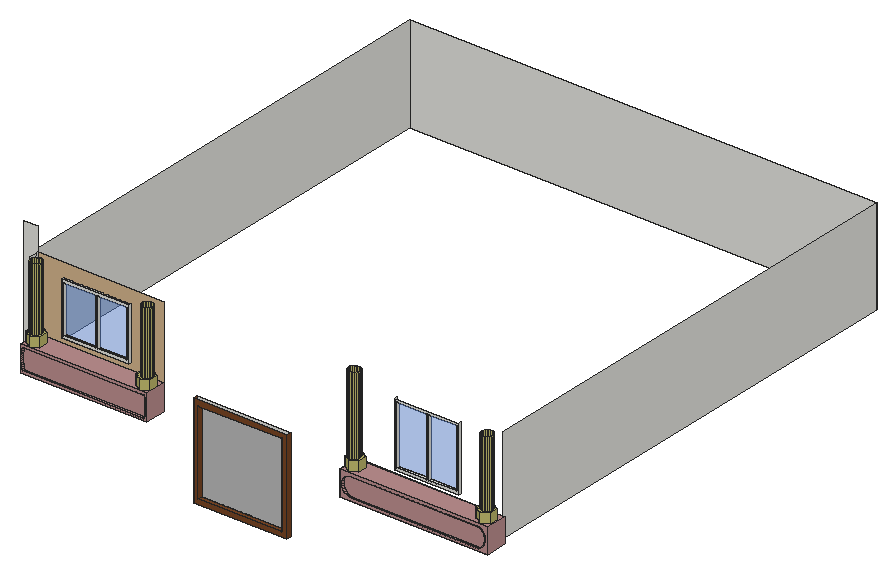
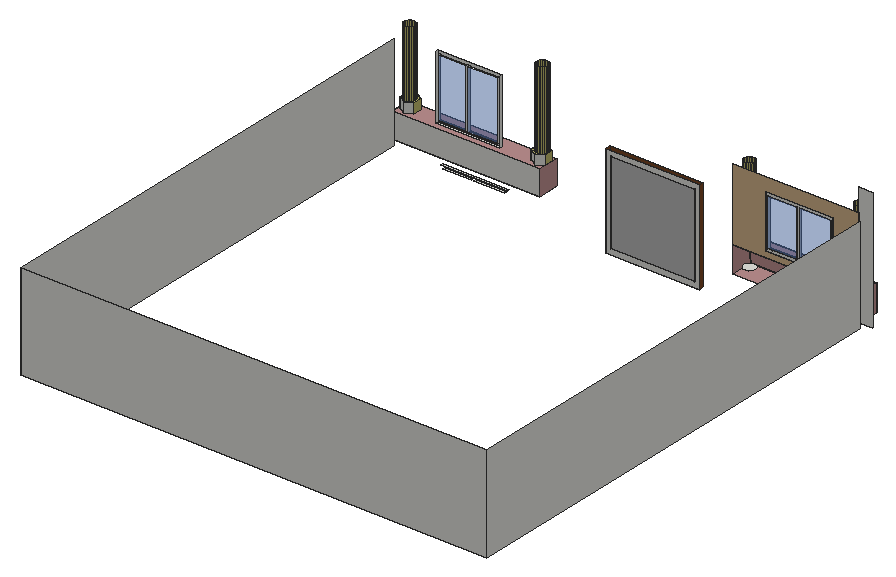
# SketchUp Ruby script. Lengths in inches.
U = 1.inch
M = Sketchup.active_model
def pt(a) = Geom::Point3d.new(a.map { |v| v * U })
def face(e, loops, mat)
  f = e.add_face(loops[0].map { |a| pt(a) })
  loops[1..].each { |l| e.add_face(l.map { |a| pt(a) }).erase! }
  f.material = f.back_material = mat if mat
  f
end
# faces: each face lists its corners as indices into pts; further lists are holes
def faces(e, pts, list, mat = nil) = list.each { |f| face(e, (f[0].is_a?(Array) ? f : [f]).map { |l| l.map { |i| pts[i] } }, mat) }
# xy, xz, yz: faces in a plane at the given z, y or x. An outline is a flat list of corners, or four numbers for a rectangle; further outlines are holes
def ring(l) = l.size == 4 ? [[l[0], l[1]], [l[2], l[1]], [l[2], l[3]], [l[0], l[3]]] : l.each_slice(2).to_a
def flat(e, list, mat, &to3) = list.each { |f| face(e, (f[0].is_a?(Array) ? f : [f]).map { |l| ring(l).map { |u, v| to3.(u, v) } }, mat) }
def xy(e, z, list, mat = nil) = flat(e, list, mat) { |x, y| [x, y, z] }
def xz(e, y, list, mat = nil) = flat(e, list, mat) { |x, z| [x, y, z] }
def yz(e, x, list, mat = nil) = flat(e, list, mat) { |y, z| [x, y, z] }
def lines(e, pts, list) = list.each { |a, b| e.add_line(pt(pts[a]), pt(pts[b])) }
# prism: a flat outline (further loops are holes) pulled along v
def prism(e, loops, v, mat = nil)
  f = face(e, loops, mat); d = Geom::Vector3d.new(v.map { |x| x * U })
  f.pushpull(f.normal.samedirection?(d) ? d.length : -d.length)
end
def box(e, o, s, mat = nil) = prism(e, [[o, [o[0] + s[0], o[1], o[2]], [o[0] + s[0], o[1] + s[1], o[2]], [o[0], o[1] + s[1], o[2]]]], [0, 0, s[2]], mat)
def at(x, y, z, deg = 0) = Geom::Transformation.translation(pt([x, y, z])) * Geom::Transformation.rotation(ORIGIN, Z_AXIS, deg.degrees)
def axes(o, x, y, z) = Geom::Transformation.new([*x, 0, *y, 0, *z, 0, *pt(o).to_a, 1])
def part(name) = M.definitions.add(name)
# library, detail: a bought-in or finely detailed component or shape, given as its bounding box
def library(name, o, s) = part(name).tap { |d| box(d.entities, o, s) }
def detail(e, o, s) = box(e.add_group.entities, o, s)
def put(e, d, t, mat = nil) = e.add_instance(d, t).tap { |i| i.material = mat if mat }
def group(e, t, mat = nil) = e.add_group.tap { |g| g.transformation = t; g.material = mat if mat }.entities
root = M.entities
M.materials.add("[0035_Tan]").color = [210, 180, 140]
M.materials.add("[0057_DarkKhaki]").color = [189, 183, 107]
M.materials.add("[0119_RosyBrown]").color = [188, 143, 143]
M.materials.add("[Mirror 01]").color = [185, 185, 185]
M.materials.add("[Translucent Glass Blue]").color = [100, 149, 237]
M.materials["[Translucent Glass Blue]"].alpha = 0.5
M.materials.add("[Wood Veneer 01]").color = [120, 70, 37]
xy(root,421.56,[[370.4,74.37,487.09,80.37]],"[Wood Veneer 01]")
xy(root,427.56,[[376.4,74.37,481.09,80.37]],"[Wood Veneer 01]")
xy(root,470.26,[[584.28,113.37,622.84,116.37],[626.17,113.37,661.4,116.37]])
xy(root,472.13,[[173.78,113.37,215.4,116.37],[217.84,113.37,257.03,116.37]])
xy(root,473.26,[[581.28,113.37,664.4,116.37]])
xy(root,475.13,[[170.78,113.37,260.03,116.37]])
xy(root,480,[[142.36,89.37,299.74,116.37]],"[0119_RosyBrown]")
xy(root,481.5,[[540.59,89.37,725.37,92.37],[540.59,92.37,725.37,116.37]],"[0119_RosyBrown]")
xy(root,483,[[145.36,89.37,296.74,92.37]],"[0119_RosyBrown]")
xy(root,484.5,[[711.84,99.06,713.26,99.24,714.59,99.79,715.73,100.67,716.6,101.81,717.15,103.13,717.34,104.56,717.15,105.98,716.6,107.31,715.73,108.44,714.59,109.32,713.26,109.87,711.84,110.06,710.41,109.87,709.09,109.32,707.95,108.44,707.07,107.31,706.53,105.98,706.34,104.56,706.53,103.13,707.07,101.81,707.95,100.67,709.09,99.79,710.41,99.24],[549.01,99.72,550.28,99.72,551.51,100.05,552.61,100.69,553.51,101.59,554.14,102.7,554.47,103.93,554.47,105.2,554.14,106.43,553.5,107.53,552.6,108.43,551.49,109.0625,550.26,109.39,548.99,109.39,547.76,109.06,546.66,108.42,545.76,107.52,545.13,106.41,544.8,105.19,544.8,103.91,545.13,102.68,545.77,101.58,546.67,100.68,547.78,100.05]])
xy(root,484.5,[[553.67,89.37,715.1,92.37]],"[0119_RosyBrown]")
xy(root,485.25,[[153.73,94.92,155.52,95.29,157.15,96.12,158.52,97.33,159.52,98.86,160.09,100.6,160.19,102.42,159.82,104.21,159,105.84,157.78,107.2,156.25,108.21,154.52,108.78,152.69,108.88,150.9,108.51,149.27,107.69,147.91,106.47,146.91,104.94,146.33,103.2,146.23,101.38,146.6,99.59,147.43,97.96,148.64,96.6,150.17,95.59,151.91,95.02],[289.98,96.17,291.77,96.54,293.4,97.37,294.77,98.58,295.77,100.11,296.34,101.85,296.44,103.67,296.07,105.46,295.25,107.09,294.03,108.45,292.5,109.46,290.77,110.03,288.94,110.13,287.15,109.76,285.52,108.94,284.16,107.72,283.16,106.19,282.58,104.45,282.48,102.63,282.85,100.84,283.68,99.21,284.89,97.85,286.42,96.84,288.16,96.27]])
xy(root,509.25,[[553.67,89.37,715.1,92.37]],"[0119_RosyBrown]")
xy(root,509.5625,[[145.36,89.37,296.74,92.37]],"[0119_RosyBrown]")
xy(root,512.25,[[[540.59,89.37,725.37,116.37],[550.07,91.65,541.14,96.81,541.14,107.12,550.07,112.27,559,107.12,559,96.81],[714.38,91.65,705.45,96.81,705.45,107.12,714.38,112.27,723.3125,107.12,723.3125,96.81]]],"[0119_RosyBrown]")
xy(root,512.5625,[[153.05,90.14,144.01,95.36,144.01,105.8,153.05,111.02,162.09,105.8,162.09,95.36],[290.49,90.14,281.45,95.36,281.45,105.8,290.49,111.02,299.53,105.8,299.53,95.36]])
xy(root,512.5625,[[[142.36,89.37,299.74,116.37],[290.49,90.14,281.45,95.36,281.45,105.8,290.49,111.02,299.53,105.8,299.53,95.36],[153.05,90.14,144.01,95.36,144.01,105.8,153.05,111.02,162.09,105.8,162.09,95.36]]],"[0119_RosyBrown]")
xy(root,518.48,[[590.68,113.37,670.37,116.37]])
xy(root,520.23,[[174.8,113.37,258.8,116.37]])
xy(root,521.48,[[593.68,113.37,630.53,116.37],[633.47,113.37,667.37,116.37]])
xy(root,523.23,[[177.8,113.37,216.8,116.37],[219.92,113.37,255.8,116.37]])
xy(root,524.25,[[[550.07,91.65,559,96.81,559,107.12,550.07,112.27,541.14,107.12,541.14,96.81],[548.88,95.41,547.09,95.64,545.41,96.33,543.98,97.4375,542.875,98.875,542.18,100.55,541.95,102.34,542.18,104.14,542.875,105.8125,543.98,107.25,545.41,108.35,547.09,109.04,548.88,109.28,550.68,109.04,552.35,108.35,553.79,107.25,554.89,105.8125,555.58,104.14,555.82,102.34,555.58,100.55,554.89,98.875,553.79,97.4375,552.35,96.33,550.68,95.64]],[[714.38,91.65,723.3125,96.81,723.3125,107.12,714.38,112.27,705.45,107.12,705.45,96.81],[714.7,95.41,712.9,95.64,711.23,96.33,709.79,97.4375,708.6875,98.875,707.99,100.55,707.76,102.34,707.99,104.14,708.6875,105.8125,709.79,107.25,711.23,108.35,712.9,109.04,714.7,109.28,716.49,109.04,718.16,108.35,719.6,107.25,720.7,105.8125,721.4,104.14,721.63,102.34,721.4,100.55,720.7,98.875,719.6,97.4375,718.16,96.33,716.49,95.64]]],"[0057_DarkKhaki]")
xy(root,524.5625,[[[153.05,90.14,162.09,95.36,162.09,105.8,153.05,111.02,144.01,105.8,144.01,95.36],[152.5,94.42,150.78,94.71,149.19,95.4375,147.84,96.55,146.83,97.97,146.22,99.61,146.06,101.35,146.35,103.07,147.07,104.66,148.18,106,149.61,107.01,151.24,107.625,152.98,107.79,154.7,107.5,156.29,106.77,157.64,105.66,158.65,104.24,159.26,102.6,159.42,100.87,159.13,99.14,158.41,97.56,157.3,96.21,155.875,95.2,154.24,94.59]],[[290.49,90.14,299.53,95.36,299.53,105.8,290.49,111.02,281.45,105.8,281.45,95.36],[291.4,94.48,289.68,94.66,288.07,95.28,286.67,96.3,285.58,97.65,284.88,99.23,284.61,100.93,284.79,102.65,285.41,104.27,286.42,105.67,287.77,106.76,289.35,107.46,291.06,107.73,292.78,107.55,294.39,106.93,295.79,105.91,296.88,104.57,297.58,102.99,297.85,101.28,297.67,99.56,297.05,97.95,296.04,96.55,294.69,95.46,293.11,94.75]]],"[0057_DarkKhaki]")
xz(root,74.37,[[[370.4,421.56,487.09,538.24],[376.4,427.56,481.09,532.24]]],"[Wood Veneer 01]")
xz(root,80.37,[[[370.4,421.56,487.09,538.24],[376.4,427.56,481.09,532.24]]])
xz(root,80.37,[[376.4,427.56,481.09,532.24]],"[Mirror 01]")
xz(root,89.37,[[[142.36,480,299.74,512.5625],[145.36,483,144.76,485.16,144.26,487.35,143.87,489.57,143.59,491.79,143.42,494.04,143.36,496.28,143.42,498.53,143.59,500.77,143.87,503,144.26,505.21,144.76,507.4,145.36,509.5625,296.74,509.5625,297.22,507.38,297.61,505.18,297.91,502.97,298.13,500.74,298.26,498.51,298.3,496.28,298.26,494.05,298.13,491.82,297.91,489.59,297.61,487.38,297.22,485.18,296.74,483]],[[540.59,481.5,725.37,512.25],[553.67,484.5,550.9375,485.4,548.48,486.89,546.43,488.9,544.88,491.32,543.92,494.02,543.59,496.875,543.92,499.73,544.88,502.43,546.43,504.85,548.48,506.86,550.9375,508.35,553.67,509.25,715.1,509.25,717.17,507.84,718.96,506.09,720.42,504.05,721.49,501.79,722.15,499.37,722.37,496.875,722.15,494.38,721.49,491.96,720.42,489.7,718.96,487.66,717.17,485.91,715.1,484.5]]],"[0119_RosyBrown]")
xz(root,92.37,[[145.36,483,296.74,483,297.22,485.18,297.61,487.38,297.91,489.59,298.13,491.82,298.26,494.05,298.3,496.28,298.26,498.51,298.13,500.74,297.91,502.97,297.61,505.18,297.22,507.38,296.74,509.5625,145.36,509.5625,144.76,507.4,144.26,505.21,143.87,503,143.59,500.77,143.42,498.53,143.36,496.28,143.42,494.04,143.59,491.79,143.87,489.57,144.26,487.35,144.76,485.16],[553.67,484.5,715.1,484.5,717.17,485.91,718.96,487.66,720.42,489.7,721.49,491.96,722.15,494.38,722.37,496.875,722.15,499.37,721.49,501.79,720.42,504.05,718.96,506.09,717.17,507.84,715.1,509.25,553.67,509.25,550.9375,508.35,548.48,506.86,546.43,504.85,544.88,502.43,543.92,499.73,543.59,496.875,543.92,494.02,544.88,491.32,546.43,488.9,548.48,486.89,550.9375,485.4]],"[0119_RosyBrown]")
xz(root,113.37,[[[590.68,518.48,670.37,598.17],[593.68,521.48,630.53,595.17],[633.47,521.48,667.37,595.17]],[[174.8,520.23,258.8,585.67],[177.8,523.23,216.8,582.67],[219.92,523.23,255.8,582.67]]])
xz(root,116.37,[[125.37,480,142.36,632],[540.59,481.5,725.37,512.25],[[174.8,520.23,258.8,585.67],[177.8,523.23,216.8,582.67],[219.92,523.23,255.8,582.67]]])
xz(root,116.37,[[[142.36,512.5625,299.74,602.86],[174.8,520.23,258.8,585.67]]],"[0035_Tan]")
xz(root,116.37,[[593.68,521.48,630.53,595.17],[633.47,521.48,667.37,595.17],[177.8,523.23,216.8,582.67],[219.92,523.23,255.8,582.67]],"[Translucent Glass Blue]")
xz(root,707.37,[[134.37,480,716.37,600]])
yz(root,134.37,[[125.37,480,707.37,600]])
yz(root,142.36,[[104.37,480,113.37,512.5625],[113.37,480,116.37,512.5625],[104.37,512.5625,113.37,602.86],[113.37,512.5625,116.37,602.86]])
yz(root,142.36,[[89.37,480,104.37,512.5625]],"[0119_RosyBrown]")
yz(root,144.01,[[95.36,512.5625,105.8,524.5625]],"[0057_DarkKhaki]")
yz(root,162.09,[[95.36,512.5625,105.8,524.5625]],"[0057_DarkKhaki]")
yz(root,174.8,[[113.37,520.23,116.37,585.67]])
yz(root,177.8,[[113.37,523.23,116.37,582.67]])
yz(root,216.8,[[113.37,523.23,116.37,582.67]])
yz(root,219.92,[[113.37,523.23,116.37,582.67]])
yz(root,255.8,[[113.37,523.23,116.37,582.67]])
yz(root,258.8,[[113.37,520.23,116.37,585.67]])
yz(root,281.45,[[95.36,512.5625,105.8,524.5625]],"[0057_DarkKhaki]")
yz(root,299.53,[[95.36,512.5625,105.8,524.5625]],"[0057_DarkKhaki]")
yz(root,299.74,[[89.37,480,116.37,512.5625]],"[0119_RosyBrown]")
yz(root,370.4,[[74.37,421.56,80.37,538.24]],"[Wood Veneer 01]")
yz(root,376.4,[[74.37,427.56,80.37,532.24]],"[Wood Veneer 01]")
yz(root,481.09,[[74.37,427.56,80.37,532.24]],"[Wood Veneer 01]")
yz(root,487.09,[[74.37,421.56,80.37,538.24]],"[Wood Veneer 01]")
yz(root,540.59,[[89.37,481.5,116.37,512.25]],"[0119_RosyBrown]")
yz(root,541.14,[[96.81,512.25,107.12,524.25]],"[0057_DarkKhaki]")
yz(root,559,[[96.81,512.25,107.12,524.25]],"[0057_DarkKhaki]")
yz(root,590.68,[[113.37,518.48,116.37,598.17]])
yz(root,593.68,[[113.37,521.48,116.37,595.17]])
yz(root,630.53,[[113.37,521.48,116.37,595.17]])
yz(root,633.47,[[113.37,521.48,116.37,595.17]])
yz(root,667.37,[[113.37,521.48,116.37,595.17]])
yz(root,670.37,[[113.37,518.48,116.37,598.17]])
yz(root,705.45,[[96.81,512.25,107.12,524.25]],"[0057_DarkKhaki]")
yz(root,716.37,[[125.37,480,707.37,600]])
yz(root,723.3125,[[96.81,512.25,107.12,524.25]],"[0057_DarkKhaki]")
yz(root,725.37,[[89.37,481.5,116.37,512.25]],"[0119_RosyBrown]")
p = [[145.36,92.37,483],[144.76,92.37,485.16],[144.76,89.37,485.16],[145.36,89.37,483],[297.22,92.37,485.18],[296.74,92.37,483],
  [296.74,89.37,483],[297.22,89.37,485.18],[553.67,92.37,484.5],[550.9375,92.37,485.4],[550.9375,89.37,485.4],[553.67,89.37,484.5],
  [717.17,92.37,485.91],[715.1,92.37,484.5],[715.1,89.37,484.5],[717.17,89.37,485.91],[144.26,92.37,487.35],[144.26,89.37,487.35],
  [297.61,92.37,487.38],[297.61,89.37,487.38],[548.48,92.37,486.89],[548.48,89.37,486.89],[718.96,92.37,487.66],[718.96,89.37,487.66],
  [546.43,92.37,488.9],[546.43,89.37,488.9],[143.87,92.37,489.57],[143.87,89.37,489.57],[297.91,92.37,489.59],[297.91,89.37,489.59],
  [720.42,92.37,489.7],[720.42,89.37,489.7],[544.88,92.37,491.32],[544.88,89.37,491.32],[143.59,92.37,491.79],[143.59,89.37,491.79],
  [298.13,92.37,491.82],[298.13,89.37,491.82],[721.49,92.37,491.96],[721.49,89.37,491.96],[543.92,92.37,494.02],[543.92,89.37,494.02],
  [143.42,92.37,494.04],[143.42,89.37,494.04],[298.26,92.37,494.05],[298.26,89.37,494.05],[722.15,92.37,494.38],[722.15,89.37,494.38],
  [143.36,92.37,496.28],[143.36,89.37,496.28],[298.3,92.37,496.28],[298.3,89.37,496.28],[543.59,92.37,496.875],[543.59,89.37,496.875],
  [722.37,92.37,496.875],[722.37,89.37,496.875],[143.42,92.37,498.53],[143.42,89.37,498.53],[298.26,92.37,498.51],[298.26,89.37,498.51],
  [543.92,92.37,499.73],[543.92,89.37,499.73],[722.15,92.37,499.37],[722.15,89.37,499.37],[143.59,92.37,500.77],[143.59,89.37,500.77],
  [298.13,92.37,500.74],[298.13,89.37,500.74],[721.49,92.37,501.79],[721.49,89.37,501.79],[544.88,92.37,502.43],[544.88,89.37,502.43],
  [297.91,92.37,502.97],[297.91,89.37,502.97],[143.87,92.37,503],[143.87,89.37,503],[720.42,92.37,504.05],[720.42,89.37,504.05],
  [546.43,92.37,504.85],[546.43,89.37,504.85],[144.26,92.37,505.21],[144.26,89.37,505.21],[297.61,92.37,505.18],[297.61,89.37,505.18],
  [718.96,92.37,506.09],[718.96,89.37,506.09],[548.48,92.37,506.86],[548.48,89.37,506.86],[144.76,92.37,507.4],[144.76,89.37,507.4],
  [297.22,92.37,507.38],[297.22,89.37,507.38],[717.17,92.37,507.84],[717.17,89.37,507.84],[550.9375,92.37,508.35],[550.9375,89.37,508.35],
  [145.36,92.37,509.5625],[145.36,89.37,509.5625],[296.74,92.37,509.5625],[296.74,89.37,509.5625],[715.1,92.37,509.25],[715.1,89.37,509.25],
  [553.67,92.37,509.25],[553.67,89.37,509.25],[541.14,96.81,512.25],[550.07,91.65,512.25],[550.07,91.65,524.25],[541.14,96.81,524.25],
  [559,96.81,512.25],[559,96.81,524.25],[705.45,96.81,512.25],[714.38,91.65,512.25],[714.38,91.65,524.25],[705.45,96.81,524.25],
  [723.3125,96.81,512.25],[723.3125,96.81,524.25],[550.07,112.27,512.25],[541.14,107.12,512.25],[541.14,107.12,524.25],[550.07,112.27,524.25],
  [559,107.12,512.25],[559,107.12,524.25],[714.38,112.27,512.25],[705.45,107.12,512.25],[705.45,107.12,524.25],[714.38,112.27,524.25],
  [723.3125,107.12,512.25],[723.3125,107.12,524.25],[144.01,95.36,512.5625],[153.05,90.14,512.5625],[153.05,90.14,524.5625],[144.01,95.36,524.5625],
  [162.09,95.36,512.5625],[162.09,95.36,524.5625],[281.45,95.36,512.5625],[290.49,90.14,512.5625],[290.49,90.14,524.5625],[281.45,95.36,524.5625],
  [299.53,95.36,512.5625],[299.53,95.36,524.5625],[153.05,111.02,512.5625],[144.01,105.8,512.5625],[144.01,105.8,524.5625],[153.05,111.02,524.5625],
  [162.09,105.8,512.5625],[162.09,105.8,524.5625],[290.49,111.02,512.5625],[281.45,105.8,512.5625],[281.45,105.8,524.5625],[290.49,111.02,524.5625],
  [299.53,105.8,512.5625],[299.53,105.8,524.5625],[547.09,95.64,524.25],[548.88,95.41,524.25],[548.88,95.41,621.125],[547.09,95.64,621.125],
  [550.68,95.64,524.25],[550.68,95.64,621.125],[712.9,95.64,524.25],[714.7,95.41,524.25],[714.7,95.41,607.5],[712.9,95.64,607.5],
  [716.49,95.64,524.25],[716.49,95.64,607.5],[545.41,96.33,524.25],[545.41,96.33,621.125],[552.35,96.33,524.25],[552.35,96.33,621.125],
  [711.23,96.33,524.25],[711.23,96.33,607.5],[718.16,96.33,524.25],[718.16,96.33,607.5],[543.98,97.4375,524.25],[543.98,97.4375,621.125],
  [553.79,97.4375,524.25],[553.79,97.4375,621.125],[709.79,97.4375,524.25],[709.79,97.4375,607.5],[719.6,97.4375,524.25],[719.6,97.4375,607.5],
  [542.875,98.875,524.25],[542.875,98.875,621.125],[554.89,98.875,524.25],[554.89,98.875,621.125],[708.6875,98.875,524.25],[708.6875,98.875,607.5],
  [720.7,98.875,524.25],[720.7,98.875,607.5],[542.18,100.55,524.25],[542.18,100.55,621.125],[555.58,100.55,524.25],[555.58,100.55,621.125],
  [707.99,100.55,524.25],[707.99,100.55,607.5],[721.4,100.55,524.25],[721.4,100.55,607.5],[541.95,102.34,524.25],[541.95,102.34,621.125],
  [555.82,102.34,524.25],[555.82,102.34,621.125],[707.76,102.34,524.25],[707.76,102.34,607.5],[721.63,102.34,524.25],[721.63,102.34,607.5],
  [542.18,104.14,524.25],[542.18,104.14,621.125],[555.58,104.14,524.25],[555.58,104.14,621.125],[707.99,104.14,524.25],[707.99,104.14,607.5],
  [721.4,104.14,524.25],[721.4,104.14,607.5],[542.875,105.8125,524.25],[542.875,105.8125,621.125],[554.89,105.8125,524.25],[554.89,105.8125,621.125],
  [708.6875,105.8125,524.25],[708.6875,105.8125,607.5],[720.7,105.8125,524.25],[720.7,105.8125,607.5],[543.98,107.25,524.25],[543.98,107.25,621.125],
  [553.79,107.25,524.25],[553.79,107.25,621.125],[709.79,107.25,524.25],[709.79,107.25,607.5],[719.6,107.25,524.25],[719.6,107.25,607.5],
  [545.41,108.35,524.25],[545.41,108.35,621.125],[552.35,108.35,524.25],[552.35,108.35,621.125],[711.23,108.35,524.25],[711.23,108.35,607.5],
  [718.16,108.35,524.25],[718.16,108.35,607.5],[547.09,109.04,524.25],[547.09,109.04,621.125],[550.68,109.04,524.25],[550.68,109.04,621.125],
  [712.9,109.04,524.25],[712.9,109.04,607.5],[716.49,109.04,524.25],[716.49,109.04,607.5],[548.88,109.28,524.25],[548.88,109.28,621.125],
  [714.7,109.28,524.25],[714.7,109.28,607.5],[150.78,94.71,524.5625],[152.5,94.42,524.5625],[152.5,94.42,603.5],[150.78,94.71,603.5],
  [154.24,94.59,524.5625],[154.24,94.59,603.5],[289.68,94.66,524.5625],[291.4,94.48,524.5625],[291.4,94.48,603.1875],[289.68,94.66,603.1875],
  [293.11,94.75,524.5625],[293.11,94.75,603.1875],[155.875,95.2,524.5625],[155.875,95.2,603.5],[149.19,95.4375,524.5625],[149.19,95.4375,603.5],
  [288.07,95.28,524.5625],[288.07,95.28,603.1875],[294.69,95.46,524.5625],[294.69,95.46,603.1875],[157.3,96.21,524.5625],[157.3,96.21,603.5],
  [286.67,96.3,524.5625],[286.67,96.3,603.1875],[147.84,96.55,524.5625],[147.84,96.55,603.5],[296.04,96.55,524.5625],[296.04,96.55,603.1875],
  [158.41,97.56,524.5625],[158.41,97.56,603.5],[285.58,97.65,524.5625],[285.58,97.65,603.1875],[297.05,97.95,524.5625],[297.05,97.95,603.1875],
  [146.83,97.97,524.5625],[146.83,97.97,603.5],[159.13,99.14,524.5625],[159.13,99.14,603.5],[284.88,99.23,524.5625],[284.88,99.23,603.1875],
  [297.67,99.56,524.5625],[297.67,99.56,603.1875],[146.22,99.61,524.5625],[146.22,99.61,603.5],[159.42,100.87,524.5625],[159.42,100.87,603.5],
  [284.61,100.93,524.5625],[284.61,100.93,603.1875],[146.06,101.35,524.5625],[146.06,101.35,603.5],[297.85,101.28,524.5625],[297.85,101.28,603.1875],
  [159.26,102.6,524.5625],[159.26,102.6,603.5],[284.79,102.65,524.5625],[284.79,102.65,603.1875],[146.35,103.07,524.5625],[146.35,103.07,603.5],
  [297.58,102.99,524.5625],[297.58,102.99,603.1875],[158.65,104.24,524.5625],[158.65,104.24,603.5],[285.41,104.27,524.5625],[285.41,104.27,603.1875],
  [296.88,104.57,524.5625],[296.88,104.57,603.1875],[147.07,104.66,524.5625],[147.07,104.66,603.5],[157.64,105.66,524.5625],[157.64,105.66,603.5],
  [286.42,105.67,524.5625],[286.42,105.67,603.1875],[295.79,105.91,524.5625],[295.79,105.91,603.1875],[148.18,106,524.5625],[148.18,106,603.5],
  [156.29,106.77,524.5625],[156.29,106.77,603.5],[287.77,106.76,524.5625],[287.77,106.76,603.1875],[294.39,106.93,524.5625],[294.39,106.93,603.1875],
  [149.61,107.01,524.5625],[149.61,107.01,603.5],[154.7,107.5,524.5625],[154.7,107.5,603.5],[289.35,107.46,524.5625],[289.35,107.46,603.1875],
  [292.78,107.55,524.5625],[292.78,107.55,603.1875],[151.24,107.625,524.5625],[151.24,107.625,603.5],[152.98,107.79,524.5625],[152.98,107.79,603.5],
  [291.06,107.73,524.5625],[291.06,107.73,603.1875]]
faces(root,p,[[0,1,2,3],[4,5,6,7],[8,9,10,11],[12,13,14,15],[1,16,17,2],[18,4,7,19],[9,20,21,10],[22,12,15,23],
  [20,24,25,21],[16,26,27,17],[28,18,19,29],[30,22,23,31],[24,32,33,25],[26,34,35,27],[36,28,29,37],[38,30,31,39],
  [32,40,41,33],[34,42,43,35],[44,36,37,45],[46,38,39,47],[42,48,49,43],[50,44,45,51],[40,52,53,41],[54,46,47,55],
  [48,56,57,49],[58,50,51,59],[52,60,61,53],[62,54,55,63],[56,64,65,57],[66,58,59,67],[68,62,63,69],[60,70,71,61],
  [72,66,67,73],[64,74,75,65],[76,68,69,77],[70,78,79,71],[74,80,81,75],[82,72,73,83],[84,76,77,85],[78,86,87,79],
  [80,88,89,81],[90,82,83,91],[92,84,85,93],[86,94,95,87],[88,96,97,89],[98,90,91,99],[100,92,93,101],[94,102,103,95]],"[0119_RosyBrown]")
faces(root,p,[[104,105,106,107],[105,108,109,106],[110,111,112,113],[111,114,115,112],[128,129,130,131],[129,132,133,130],[134,135,136,137],[135,138,139,136],
  [152,153,154,155],[153,156,157,154],[158,159,160,161],[159,162,163,160],[164,152,155,165],[156,166,167,157],[168,158,161,169],[162,170,171,163],
  [172,164,165,173],[166,174,175,167],[176,168,169,177],[170,178,179,171],[180,172,173,181],[174,182,183,175],[184,176,177,185],[178,186,187,179],
  [188,180,181,189],[182,190,191,183],[192,184,185,193],[186,194,195,187],[196,188,189,197],[190,198,199,191],[200,192,193,201],[194,202,203,195],
  [204,196,197,205],[198,206,207,199],[208,200,201,209],[202,210,211,203],[212,204,205,213],[206,214,215,207],[216,208,209,217],[210,218,219,211],
  [220,212,213,221],[214,222,223,215],[224,216,217,225],[218,226,227,219],[228,220,221,229],[222,230,231,223],[232,224,225,233],[226,234,235,227],
  [236,228,229,237],[230,238,239,231],[240,232,233,241],[234,242,243,235],[244,236,237,245],[238,244,245,239],[246,240,241,247],[242,246,247,243],
  [248,249,250,251],[249,252,253,250],[254,255,256,257],[255,258,259,256],[252,260,261,253],[262,248,251,263],[264,254,257,265],[258,266,267,259],
  [260,268,269,261],[270,264,265,271],[272,262,263,273],[266,274,275,267],[268,276,277,269],[278,270,271,279],[274,280,281,275],[282,272,273,283],
  [276,284,285,277],[286,278,279,287],[280,288,289,281],[290,282,283,291],[284,292,293,285],[294,286,287,295],[296,290,291,297],[288,298,299,289],
  [292,300,301,293],[302,294,295,303],[304,296,297,305],[298,306,307,299],[300,308,309,301],[310,302,303,311],[306,312,313,307],[314,304,305,315],
  [308,316,317,309],[318,310,311,319],[312,320,321,313],[322,314,315,323],[316,324,325,317],[326,318,319,327],[320,328,329,321],[330,322,323,331],
  [324,332,333,325],[334,326,327,335],[328,336,337,329],[338,330,331,339],[332,340,341,333],[342,334,335,343],[336,342,343,337],[340,338,339,341]],"[0057_DarkKhaki]")
faces(root,p,[[116,117,118,119],[120,116,119,121],[122,123,124,125],[126,122,125,127],[140,141,142,143],[144,140,143,145],[146,147,148,149],[150,146,149,151]])
